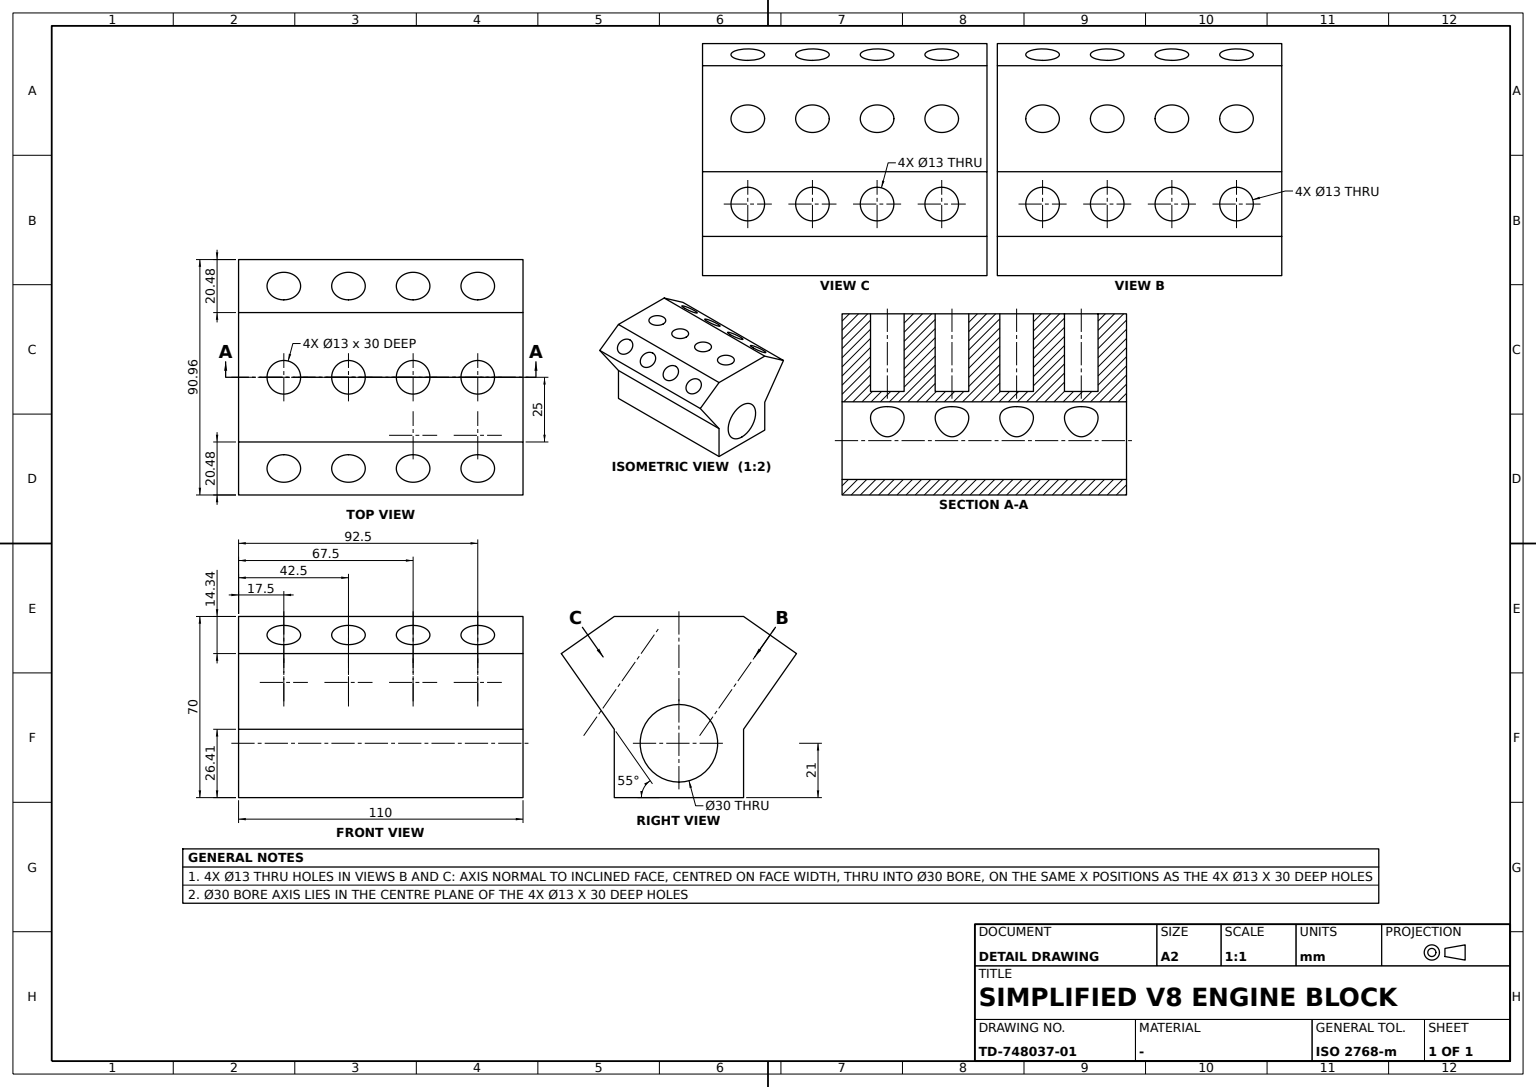
ISO-10303-21;
HEADER;
FILE_DESCRIPTION((''),'2;1');
FILE_NAME('','',(''),(''),'','','');
FILE_SCHEMA(('AUTOMOTIVE_DESIGN'));
ENDSEC;
DATA;
#1=APPLICATION_CONTEXT('');
#2=PRODUCT_CONTEXT('',#1,'mechanical');
#3=PRODUCT('','','',(#2));
#4=PRODUCT_DEFINITION_FORMATION('','',#3);
#5=PRODUCT_DEFINITION_CONTEXT('',#1,'design');
#6=PRODUCT_DEFINITION('','',#4,#5);
#7=PRODUCT_DEFINITION_SHAPE('','',#6);
#8=(LENGTH_UNIT()NAMED_UNIT(*)SI_UNIT(.MILLI.,.METRE.));
#9=(NAMED_UNIT(*)PLANE_ANGLE_UNIT()SI_UNIT($,.RADIAN.));
#10=(NAMED_UNIT(*)SI_UNIT($,.STERADIAN.)SOLID_ANGLE_UNIT());
#11=UNCERTAINTY_MEASURE_WITH_UNIT(LENGTH_MEASURE(0.005),#8,'distance_accuracy_value','');
#12=(GEOMETRIC_REPRESENTATION_CONTEXT(3)GLOBAL_UNCERTAINTY_ASSIGNED_CONTEXT((#11))GLOBAL_UNIT_ASSIGNED_CONTEXT((#8,#9,#10))REPRESENTATION_CONTEXT('',''));
#13=CARTESIAN_POINT('',(11.,-12.129513,29.824676));
#14=VERTEX_POINT('',#13);
#15=CARTESIAN_POINT('',(11.331638,-13.567226,27.566825));
#16=CARTESIAN_POINT('',(10.831406,-12.200834,29.868851));
#17=CARTESIAN_POINT('',(11.342736,-10.406518,31.905828));
#18=CARTESIAN_POINT('',(13.425697,-8.035123,33.778753));
#19=CARTESIAN_POINT('',(18.017567,-6.520434,34.487409));
#20=CARTESIAN_POINT('',(22.326173,-8.58199,33.456222));
#21=CARTESIAN_POINT('',(23.956477,-11.040954,31.272985));
#22=CARTESIAN_POINT('',(24.098074,-12.732658,29.08519));
#23=CARTESIAN_POINT('',(23.306824,-13.919542,26.765346));
#24=CARTESIAN_POINT('',(21.825814,-14.611855,24.598701));
#25=CARTESIAN_POINT('',(19.755642,-14.903136,22.838252));
#26=CARTESIAN_POINT('',(16.99593,-14.94974,22.2127));
#27=CARTESIAN_POINT('',(14.451282,-14.839464,23.383385));
#28=CARTESIAN_POINT('',(12.594119,-14.423445,25.313733));
#29=B_SPLINE_CURVE_WITH_KNOTS('',3,(#15,#16,#17,#18,#19,#20,#21,#22,#23,#24,#25,#26,#27,#28,#15,#16,#17),.UNSPECIFIED.,.T.,.F.,(1,1,1,1,1,1,1,1,1,1,1,1,1,1,1,1,1,1,1,1,1),(-0.008032053,-0.005354702,-0.002677351,0.,0.002677351,0.005354702,0.010709404,0.016064107,0.018741458,0.021418809,0.02409616,0.026773511,0.029450862,0.032128213,0.034805564,0.037482915,0.040160267,0.042837618,0.045514969,0.04819232,0.053547022),.UNSPECIFIED.);
#30=EDGE_CURVE('',#14,#14,#29,.T.);
#31=ORIENTED_EDGE('',*,*,#30,.T.);
#32=EDGE_LOOP('',(#31));
#33=FACE_BOUND('',#32,.T.);
#34=CARTESIAN_POINT('',(17.5,-29.914912,66.557263));
#35=VERTEX_POINT('',#34);
#36=CARTESIAN_POINT('',(17.5,-35.239401,62.829016));
#37=DIRECTION('',(0.,0.573576436,-0.819152044));
#38=DIRECTION('',(0.,0.819152044,0.573576436));
#39=AXIS2_PLACEMENT_3D('',#36,#37,#38);
#40=CIRCLE('',#39,6.5);
#41=EDGE_CURVE('',#35,#35,#40,.T.);
#42=ORIENTED_EDGE('',*,*,#41,.F.);
#43=EDGE_LOOP('',(#42));
#44=FACE_BOUND('',#43,.T.);
#45=CARTESIAN_POINT('',(17.5,-3.283467,17.191213));
#46=DIRECTION('',(-1.,0.,0.));
#47=AXIS2_PLACEMENT_3D('',#45,#37,#46);
#48=CYLINDRICAL_SURFACE('',#47,6.5);
#49=ADVANCED_FACE('',(#33,#44),#48,.F.);
#50=CARTESIAN_POINT('',(24.,12.129513,29.824676));
#51=VERTEX_POINT('',#50);
#52=CARTESIAN_POINT('',(23.655254,10.402376,31.909925));
#53=CARTESIAN_POINT('',(24.169445,12.201153,29.869133));
#54=CARTESIAN_POINT('',(23.666966,13.570089,27.561601));
#55=CARTESIAN_POINT('',(22.399301,14.425934,25.305088));
#56=CARTESIAN_POINT('',(20.543939,14.839822,23.379841));
#57=CARTESIAN_POINT('',(17.996344,14.949835,22.211813));
#58=CARTESIAN_POINT('',(15.240789,14.902833,22.841055));
#59=CARTESIAN_POINT('',(13.173241,14.611379,24.600066));
#60=CARTESIAN_POINT('',(11.692868,13.919632,26.765493));
#61=CARTESIAN_POINT('',(10.904365,12.732991,29.082723));
#62=CARTESIAN_POINT('',(11.037993,11.056515,31.256057));
#63=CARTESIAN_POINT('',(12.666972,8.58389,33.457391));
#64=CARTESIAN_POINT('',(16.974637,6.521635,34.486021));
#65=CARTESIAN_POINT('',(21.569199,8.031851,33.78052));
#66=B_SPLINE_CURVE_WITH_KNOTS('',3,(#52,#53,#54,#55,#56,#57,#58,#59,#60,#61,#62,#63,#64,#65,#52,#53,#54),.UNSPECIFIED.,.T.,.F.,(1,1,1,1,1,1,1,1,1,1,1,1,1,1,1,1,1,1,1,1,1),(-0.010684726,-0.005342363,-0.002671181,0.,0.002671181,0.005342363,0.008013544,0.010684726,0.013355907,0.016027089,0.01869827,0.021369452,0.024040633,0.026711815,0.032054178,0.037396541,0.040067722,0.042738904,0.045410085,0.048081267,0.050752448),.UNSPECIFIED.);
#67=EDGE_CURVE('',#51,#51,#66,.T.);
#68=ORIENTED_EDGE('',*,*,#67,.F.);
#69=EDGE_LOOP('',(#68));
#70=FACE_BOUND('',#69,.T.);
#71=CARTESIAN_POINT('',(17.5,29.914912,66.557263));
#72=VERTEX_POINT('',#71);
#73=CARTESIAN_POINT('',(17.5,35.239401,62.829016));
#74=DIRECTION('',(0.,0.573576436,0.819152044));
#75=DIRECTION('',(0.,-0.819152044,0.573576436));
#76=AXIS2_PLACEMENT_3D('',#73,#74,#75);
#77=CIRCLE('',#76,6.5);
#78=EDGE_CURVE('',#72,#72,#77,.T.);
#79=ORIENTED_EDGE('',*,*,#78,.T.);
#80=EDGE_LOOP('',(#79));
#81=FACE_BOUND('',#80,.T.);
#82=CARTESIAN_POINT('',(17.5,3.283467,17.191213));
#83=AXIS2_PLACEMENT_3D('',#82,#74,#46);
#84=CYLINDRICAL_SURFACE('',#83,6.5);
#85=ADVANCED_FACE('',(#70,#81),#84,.F.);
#86=CARTESIAN_POINT('',(24.,0.,39.998722));
#87=VERTEX_POINT('',#86);
#88=CARTESIAN_POINT('',(17.5,0.,39.998722));
#89=DIRECTION('',(0.,0.,1.));
#90=DIRECTION('',(1.,0.,0.));
#91=AXIS2_PLACEMENT_3D('',#88,#89,#90);
#92=CIRCLE('',#91,6.5);
#93=EDGE_CURVE('',#87,#87,#92,.T.);
#94=ORIENTED_EDGE('',*,*,#93,.T.);
#95=EDGE_LOOP('',(#94));
#96=FACE_BOUND('',#95,.T.);
#97=CARTESIAN_POINT('',(0.,0.,39.998722));
#98=AXIS2_PLACEMENT_3D('',#97,#89,#90);
#99=PLANE('',#98);
#100=ADVANCED_FACE('',(#96),#99,.T.);
#101=CARTESIAN_POINT('',(86.,0.,69.998722));
#102=VERTEX_POINT('',#101);
#103=CARTESIAN_POINT('',(92.5,0.,69.998722));
#104=DIRECTION('',(0.,0.,-1.));
#105=AXIS2_PLACEMENT_3D('',#103,#104,#46);
#106=CIRCLE('',#105,6.5);
#107=EDGE_CURVE('',#102,#102,#106,.F.);
#108=ORIENTED_EDGE('',*,*,#107,.T.);
#109=EDGE_LOOP('',(#108));
#110=FACE_BOUND('',#109,.T.);
#111=CARTESIAN_POINT('',(99.,0.,39.998722));
#112=VERTEX_POINT('',#111);
#113=CARTESIAN_POINT('',(92.5,0.,39.998722));
#114=AXIS2_PLACEMENT_3D('',#113,#89,#90);
#115=CIRCLE('',#114,6.5);
#116=EDGE_CURVE('',#112,#112,#115,.T.);
#117=ORIENTED_EDGE('',*,*,#116,.F.);
#118=EDGE_LOOP('',(#117));
#119=FACE_BOUND('',#118,.T.);
#120=CARTESIAN_POINT('',(92.5,0.,54.998722));
#121=AXIS2_PLACEMENT_3D('',#120,#89,#90);
#122=CYLINDRICAL_SURFACE('',#121,6.5);
#123=ADVANCED_FACE('',(#110,#119),#122,.F.);
#124=CARTESIAN_POINT('',(36.,-12.129513,29.824676));
#125=VERTEX_POINT('',#124);
#126=CARTESIAN_POINT('',(36.331638,-13.567226,27.566825));
#127=CARTESIAN_POINT('',(35.831406,-12.200834,29.868851));
#128=CARTESIAN_POINT('',(36.342736,-10.406518,31.905828));
#129=CARTESIAN_POINT('',(38.425697,-8.035123,33.778753));
#130=CARTESIAN_POINT('',(43.017567,-6.520434,34.487409));
#131=CARTESIAN_POINT('',(47.326173,-8.58199,33.456222));
#132=CARTESIAN_POINT('',(48.956477,-11.040954,31.272985));
#133=CARTESIAN_POINT('',(49.098074,-12.732658,29.08519));
#134=CARTESIAN_POINT('',(48.306824,-13.919542,26.765346));
#135=CARTESIAN_POINT('',(46.825814,-14.611855,24.598701));
#136=CARTESIAN_POINT('',(44.755642,-14.903136,22.838252));
#137=CARTESIAN_POINT('',(41.99593,-14.94974,22.2127));
#138=CARTESIAN_POINT('',(39.451282,-14.839464,23.383385));
#139=CARTESIAN_POINT('',(37.594119,-14.423445,25.313733));
#140=B_SPLINE_CURVE_WITH_KNOTS('',3,(#126,#127,#128,#129,#130,#131,#132,#133,#134,#135,#136,#137,#138,#139,#126,#127,#128),.UNSPECIFIED.,.T.,.F.,(1,1,1,1,1,1,1,1,1,1,1,1,1,1,1,1,1,1,1,1,1),(-0.008032053,-0.005354702,-0.002677351,0.,0.002677351,0.005354702,0.010709404,0.016064107,0.018741458,0.021418809,0.02409616,0.026773511,0.029450862,0.032128213,0.034805564,0.037482915,0.040160267,0.042837618,0.045514969,0.04819232,0.053547022),.UNSPECIFIED.);
#141=EDGE_CURVE('',#125,#125,#140,.T.);
#142=ORIENTED_EDGE('',*,*,#141,.T.);
#143=EDGE_LOOP('',(#142));
#144=FACE_BOUND('',#143,.T.);
#145=CARTESIAN_POINT('',(42.5,-29.914912,66.557263));
#146=VERTEX_POINT('',#145);
#147=CARTESIAN_POINT('',(42.5,-35.239401,62.829016));
#148=AXIS2_PLACEMENT_3D('',#147,#37,#38);
#149=CIRCLE('',#148,6.5);
#150=EDGE_CURVE('',#146,#146,#149,.T.);
#151=ORIENTED_EDGE('',*,*,#150,.F.);
#152=EDGE_LOOP('',(#151));
#153=FACE_BOUND('',#152,.T.);
#154=CARTESIAN_POINT('',(42.5,-3.283467,17.191213));
#155=AXIS2_PLACEMENT_3D('',#154,#37,#46);
#156=CYLINDRICAL_SURFACE('',#155,6.5);
#157=ADVANCED_FACE('',(#144,#153),#156,.F.);
#158=ORIENTED_EDGE('',*,*,#41,.T.);
#159=EDGE_LOOP('',(#158));
#160=FACE_BOUND('',#159,.T.);
#161=CARTESIAN_POINT('',(0.,-45.48,55.658471));
#162=VERTEX_POINT('',#161);
#163=CARTESIAN_POINT('',(110.,-45.48,55.658471));
#164=VERTEX_POINT('',#163);
#165=VECTOR('',#90,1000.);
#166=LINE('',#161,#165);
#167=EDGE_CURVE('',#162,#164,#166,.T.);
#168=ORIENTED_EDGE('',*,*,#167,.T.);
#169=CARTESIAN_POINT('',(110.,-25.,69.998722));
#170=VERTEX_POINT('',#169);
#171=CARTESIAN_POINT('',(110.,-41.113389,58.716005));
#172=VECTOR('',#38,1000.);
#173=LINE('',#171,#172);
#174=EDGE_CURVE('',#164,#170,#173,.T.);
#175=ORIENTED_EDGE('',*,*,#174,.T.);
#176=CARTESIAN_POINT('',(0.,-25.,69.998722));
#177=VERTEX_POINT('',#176);
#178=LINE('',#176,#165);
#179=EDGE_CURVE('',#177,#170,#178,.T.);
#180=ORIENTED_EDGE('',*,*,#179,.F.);
#181=CARTESIAN_POINT('',(0.,-41.113389,58.716005));
#182=LINE('',#181,#172);
#183=EDGE_CURVE('',#162,#177,#182,.T.);
#184=ORIENTED_EDGE('',*,*,#183,.F.);
#185=EDGE_LOOP('',(#168,#175,#180,#184));
#186=FACE_BOUND('',#185,.T.);
#187=CARTESIAN_POINT('',(92.5,-29.914912,66.557263));
#188=VERTEX_POINT('',#187);
#189=CARTESIAN_POINT('',(92.5,-35.239401,62.829016));
#190=AXIS2_PLACEMENT_3D('',#189,#37,#38);
#191=CIRCLE('',#190,6.5);
#192=EDGE_CURVE('',#188,#188,#191,.T.);
#193=ORIENTED_EDGE('',*,*,#192,.T.);
#194=EDGE_LOOP('',(#193));
#195=FACE_BOUND('',#194,.T.);
#196=CARTESIAN_POINT('',(67.5,-29.914912,66.557263));
#197=VERTEX_POINT('',#196);
#198=CARTESIAN_POINT('',(67.5,-35.239401,62.829016));
#199=AXIS2_PLACEMENT_3D('',#198,#37,#38);
#200=CIRCLE('',#199,6.5);
#201=EDGE_CURVE('',#197,#197,#200,.T.);
#202=ORIENTED_EDGE('',*,*,#201,.T.);
#203=EDGE_LOOP('',(#202));
#204=FACE_BOUND('',#203,.T.);
#205=ORIENTED_EDGE('',*,*,#150,.T.);
#206=EDGE_LOOP('',(#205));
#207=FACE_BOUND('',#206,.T.);
#208=AXIS2_PLACEMENT_3D('',#161,#37,#38);
#209=PLANE('',#208);
#210=ADVANCED_FACE('',(#160,#186,#195,#204,#207),#209,.F.);
#211=ORIENTED_EDGE('',*,*,#192,.F.);
#212=EDGE_LOOP('',(#211));
#213=FACE_BOUND('',#212,.T.);
#214=CARTESIAN_POINT('',(99.,-12.129513,29.824676));
#215=VERTEX_POINT('',#214);
#216=CARTESIAN_POINT('',(98.655254,-10.402376,31.909925));
#217=CARTESIAN_POINT('',(99.169445,-12.201153,29.869133));
#218=CARTESIAN_POINT('',(98.666966,-13.570089,27.561601));
#219=CARTESIAN_POINT('',(97.399301,-14.425934,25.305088));
#220=CARTESIAN_POINT('',(95.543939,-14.839822,23.379841));
#221=CARTESIAN_POINT('',(92.996344,-14.949835,22.211813));
#222=CARTESIAN_POINT('',(90.240789,-14.902833,22.841055));
#223=CARTESIAN_POINT('',(88.173241,-14.611379,24.600066));
#224=CARTESIAN_POINT('',(86.692868,-13.919632,26.765493));
#225=CARTESIAN_POINT('',(85.904365,-12.732991,29.082723));
#226=CARTESIAN_POINT('',(86.037993,-11.056515,31.256057));
#227=CARTESIAN_POINT('',(87.666972,-8.58389,33.457391));
#228=CARTESIAN_POINT('',(91.974637,-6.521635,34.486021));
#229=CARTESIAN_POINT('',(96.569199,-8.031851,33.78052));
#230=B_SPLINE_CURVE_WITH_KNOTS('',3,(#216,#217,#218,#219,#220,#221,#222,#223,#224,#225,#226,#227,#228,#229,#216,#217,#218),.UNSPECIFIED.,.T.,.F.,(1,1,1,1,1,1,1,1,1,1,1,1,1,1,1,1,1,1,1,1,1),(-0.010684726,-0.005342363,-0.002671181,0.,0.002671181,0.005342363,0.008013544,0.010684726,0.013355907,0.016027089,0.01869827,0.021369452,0.024040633,0.026711815,0.032054178,0.037396541,0.040067722,0.042738904,0.045410085,0.048081267,0.050752448),.UNSPECIFIED.);
#231=EDGE_CURVE('',#215,#215,#230,.T.);
#232=ORIENTED_EDGE('',*,*,#231,.T.);
#233=EDGE_LOOP('',(#232));
#234=FACE_BOUND('',#233,.T.);
#235=CARTESIAN_POINT('',(92.5,-3.283467,17.191213));
#236=AXIS2_PLACEMENT_3D('',#235,#37,#46);
#237=CYLINDRICAL_SURFACE('',#236,6.5);
#238=ADVANCED_FACE('',(#213,#234),#237,.F.);
#239=ORIENTED_EDGE('',*,*,#116,.T.);
#240=EDGE_LOOP('',(#239));
#241=FACE_BOUND('',#240,.T.);
#242=ADVANCED_FACE('',(#241),#99,.T.);
#243=CARTESIAN_POINT('',(74.,0.,39.998722));
#244=VERTEX_POINT('',#243);
#245=CARTESIAN_POINT('',(67.5,0.,39.998722));
#246=AXIS2_PLACEMENT_3D('',#245,#89,#90);
#247=CIRCLE('',#246,6.5);
#248=EDGE_CURVE('',#244,#244,#247,.T.);
#249=ORIENTED_EDGE('',*,*,#248,.T.);
#250=EDGE_LOOP('',(#249));
#251=FACE_BOUND('',#250,.T.);
#252=ADVANCED_FACE('',(#251),#99,.T.);
#253=ORIENTED_EDGE('',*,*,#248,.F.);
#254=EDGE_LOOP('',(#253));
#255=FACE_BOUND('',#254,.T.);
#256=CARTESIAN_POINT('',(61.,0.,69.998722));
#257=VERTEX_POINT('',#256);
#258=CARTESIAN_POINT('',(67.5,0.,69.998722));
#259=AXIS2_PLACEMENT_3D('',#258,#104,#46);
#260=CIRCLE('',#259,6.5);
#261=EDGE_CURVE('',#257,#257,#260,.F.);
#262=ORIENTED_EDGE('',*,*,#261,.T.);
#263=EDGE_LOOP('',(#262));
#264=FACE_BOUND('',#263,.T.);
#265=CARTESIAN_POINT('',(67.5,0.,54.998722));
#266=AXIS2_PLACEMENT_3D('',#265,#89,#90);
#267=CYLINDRICAL_SURFACE('',#266,6.5);
#268=ADVANCED_FACE('',(#255,#264),#267,.F.);
#269=CARTESIAN_POINT('',(0.,25.,26.41));
#270=VERTEX_POINT('',#269);
#271=CARTESIAN_POINT('',(110.,25.,26.41));
#272=VERTEX_POINT('',#271);
#273=LINE('',#269,#165);
#274=EDGE_CURVE('',#270,#272,#273,.T.);
#275=ORIENTED_EDGE('',*,*,#274,.F.);
#276=CARTESIAN_POINT('',(0.,45.48,55.658471));
#277=VERTEX_POINT('',#276);
#278=CARTESIAN_POINT('',(0.,4.366611,-3.057534));
#279=VECTOR('',#74,1000.);
#280=LINE('',#278,#279);
#281=EDGE_CURVE('',#270,#277,#280,.T.);
#282=ORIENTED_EDGE('',*,*,#281,.T.);
#283=CARTESIAN_POINT('',(110.,45.48,55.658471));
#284=VERTEX_POINT('',#283);
#285=LINE('',#276,#165);
#286=EDGE_CURVE('',#277,#284,#285,.T.);
#287=ORIENTED_EDGE('',*,*,#286,.T.);
#288=CARTESIAN_POINT('',(110.,4.366611,-3.057534));
#289=LINE('',#288,#279);
#290=EDGE_CURVE('',#272,#284,#289,.T.);
#291=ORIENTED_EDGE('',*,*,#290,.F.);
#292=EDGE_LOOP('',(#275,#282,#287,#291));
#293=FACE_BOUND('',#292,.T.);
#294=DIRECTION('',(0.,0.819152044,-0.573576436));
#295=AXIS2_PLACEMENT_3D('',#269,#294,#74);
#296=PLANE('',#295);
#297=ADVANCED_FACE('',(#293),#296,.T.);
#298=CARTESIAN_POINT('',(110.,-25.,0.));
#299=VERTEX_POINT('',#298);
#300=CARTESIAN_POINT('',(110.,25.,0.));
#301=VERTEX_POINT('',#300);
#302=CARTESIAN_POINT('',(110.,0.,0.));
#303=DIRECTION('',(0.,1.,0.));
#304=VECTOR('',#303,1000.);
#305=LINE('',#302,#304);
#306=EDGE_CURVE('',#299,#301,#305,.T.);
#307=ORIENTED_EDGE('',*,*,#306,.F.);
#308=CARTESIAN_POINT('',(0.,-25.,0.));
#309=VERTEX_POINT('',#308);
#310=LINE('',#308,#165);
#311=EDGE_CURVE('',#309,#299,#310,.T.);
#312=ORIENTED_EDGE('',*,*,#311,.F.);
#313=CARTESIAN_POINT('',(0.,25.,0.));
#314=VERTEX_POINT('',#313);
#315=CARTESIAN_POINT('',(0.,0.,0.));
#316=LINE('',#315,#304);
#317=EDGE_CURVE('',#309,#314,#316,.T.);
#318=ORIENTED_EDGE('',*,*,#317,.T.);
#319=LINE('',#313,#165);
#320=EDGE_CURVE('',#314,#301,#319,.T.);
#321=ORIENTED_EDGE('',*,*,#320,.T.);
#322=EDGE_LOOP('',(#307,#312,#318,#321));
#323=FACE_BOUND('',#322,.T.);
#324=AXIS2_PLACEMENT_3D('',#308,#104,#303);
#325=PLANE('',#324);
#326=ADVANCED_FACE('',(#323),#325,.T.);
#327=CARTESIAN_POINT('',(49.,0.,39.998722));
#328=VERTEX_POINT('',#327);
#329=CARTESIAN_POINT('',(42.5,0.,39.998722));
#330=AXIS2_PLACEMENT_3D('',#329,#89,#90);
#331=CIRCLE('',#330,6.5);
#332=EDGE_CURVE('',#328,#328,#331,.T.);
#333=ORIENTED_EDGE('',*,*,#332,.F.);
#334=EDGE_LOOP('',(#333));
#335=FACE_BOUND('',#334,.T.);
#336=CARTESIAN_POINT('',(36.,0.,69.998722));
#337=VERTEX_POINT('',#336);
#338=CARTESIAN_POINT('',(42.5,0.,69.998722));
#339=AXIS2_PLACEMENT_3D('',#338,#104,#46);
#340=CIRCLE('',#339,6.5);
#341=EDGE_CURVE('',#337,#337,#340,.F.);
#342=ORIENTED_EDGE('',*,*,#341,.T.);
#343=EDGE_LOOP('',(#342));
#344=FACE_BOUND('',#343,.T.);
#345=CARTESIAN_POINT('',(42.5,0.,54.998722));
#346=AXIS2_PLACEMENT_3D('',#345,#89,#90);
#347=CYLINDRICAL_SURFACE('',#346,6.5);
#348=ADVANCED_FACE('',(#335,#344),#347,.F.);
#349=CARTESIAN_POINT('',(92.5,29.914912,66.557263));
#350=VERTEX_POINT('',#349);
#351=CARTESIAN_POINT('',(92.5,35.239401,62.829016));
#352=AXIS2_PLACEMENT_3D('',#351,#74,#75);
#353=CIRCLE('',#352,6.5);
#354=EDGE_CURVE('',#350,#350,#353,.T.);
#355=ORIENTED_EDGE('',*,*,#354,.T.);
#356=EDGE_LOOP('',(#355));
#357=FACE_BOUND('',#356,.T.);
#358=CARTESIAN_POINT('',(99.,12.129513,29.824676));
#359=VERTEX_POINT('',#358);
#360=CARTESIAN_POINT('',(98.655254,10.402376,31.909925));
#361=CARTESIAN_POINT('',(99.169445,12.201153,29.869133));
#362=CARTESIAN_POINT('',(98.666966,13.570089,27.561601));
#363=CARTESIAN_POINT('',(97.399301,14.425934,25.305088));
#364=CARTESIAN_POINT('',(95.543939,14.839822,23.379841));
#365=CARTESIAN_POINT('',(92.996344,14.949835,22.211813));
#366=CARTESIAN_POINT('',(90.240789,14.902833,22.841055));
#367=CARTESIAN_POINT('',(88.173241,14.611379,24.600066));
#368=CARTESIAN_POINT('',(86.692868,13.919632,26.765493));
#369=CARTESIAN_POINT('',(85.904365,12.732991,29.082723));
#370=CARTESIAN_POINT('',(86.037993,11.056515,31.256057));
#371=CARTESIAN_POINT('',(87.666972,8.58389,33.457391));
#372=CARTESIAN_POINT('',(91.974637,6.521635,34.486021));
#373=CARTESIAN_POINT('',(96.569199,8.031851,33.78052));
#374=B_SPLINE_CURVE_WITH_KNOTS('',3,(#360,#361,#362,#363,#364,#365,#366,#367,#368,#369,#370,#371,#372,#373,#360,#361,#362),.UNSPECIFIED.,.T.,.F.,(1,1,1,1,1,1,1,1,1,1,1,1,1,1,1,1,1,1,1,1,1),(-0.010684726,-0.005342363,-0.002671181,0.,0.002671181,0.005342363,0.008013544,0.010684726,0.013355907,0.016027089,0.01869827,0.021369452,0.024040633,0.026711815,0.032054178,0.037396541,0.040067722,0.042738904,0.045410085,0.048081267,0.050752448),.UNSPECIFIED.);
#375=EDGE_CURVE('',#359,#359,#374,.T.);
#376=ORIENTED_EDGE('',*,*,#375,.F.);
#377=EDGE_LOOP('',(#376));
#378=FACE_BOUND('',#377,.T.);
#379=CARTESIAN_POINT('',(92.5,3.283467,17.191213));
#380=AXIS2_PLACEMENT_3D('',#379,#74,#46);
#381=CYLINDRICAL_SURFACE('',#380,6.5);
#382=ADVANCED_FACE('',(#357,#378),#381,.F.);
#383=ORIENTED_EDGE('',*,*,#311,.T.);
#384=CARTESIAN_POINT('',(110.,-25.,26.41));
#385=VERTEX_POINT('',#384);
#386=VECTOR('',#89,1000.);
#387=LINE('',#298,#386);
#388=EDGE_CURVE('',#299,#385,#387,.T.);
#389=ORIENTED_EDGE('',*,*,#388,.T.);
#390=CARTESIAN_POINT('',(0.,-25.,26.41));
#391=VERTEX_POINT('',#390);
#392=LINE('',#390,#165);
#393=EDGE_CURVE('',#391,#385,#392,.T.);
#394=ORIENTED_EDGE('',*,*,#393,.F.);
#395=LINE('',#308,#386);
#396=EDGE_CURVE('',#309,#391,#395,.T.);
#397=ORIENTED_EDGE('',*,*,#396,.F.);
#398=EDGE_LOOP('',(#383,#389,#394,#397));
#399=FACE_BOUND('',#398,.T.);
#400=AXIS2_PLACEMENT_3D('',#308,#303,#89);
#401=PLANE('',#400);
#402=ADVANCED_FACE('',(#399),#401,.F.);
#403=ORIENTED_EDGE('',*,*,#274,.T.);
#404=LINE('',#300,#386);
#405=EDGE_CURVE('',#301,#272,#404,.T.);
#406=ORIENTED_EDGE('',*,*,#405,.F.);
#407=ORIENTED_EDGE('',*,*,#320,.F.);
#408=LINE('',#313,#386);
#409=EDGE_CURVE('',#314,#270,#408,.T.);
#410=ORIENTED_EDGE('',*,*,#409,.T.);
#411=EDGE_LOOP('',(#403,#406,#407,#410));
#412=FACE_BOUND('',#411,.T.);
#413=AXIS2_PLACEMENT_3D('',#313,#303,#89);
#414=PLANE('',#413);
#415=ADVANCED_FACE('',(#412),#414,.T.);
#416=CARTESIAN_POINT('',(74.,12.129513,29.824676));
#417=VERTEX_POINT('',#416);
#418=CARTESIAN_POINT('',(73.655254,10.402376,31.909925));
#419=CARTESIAN_POINT('',(74.169445,12.201153,29.869133));
#420=CARTESIAN_POINT('',(73.666966,13.570089,27.561601));
#421=CARTESIAN_POINT('',(72.399301,14.425934,25.305088));
#422=CARTESIAN_POINT('',(70.543939,14.839822,23.379841));
#423=CARTESIAN_POINT('',(67.996344,14.949835,22.211813));
#424=CARTESIAN_POINT('',(65.240789,14.902833,22.841055));
#425=CARTESIAN_POINT('',(63.173241,14.611379,24.600066));
#426=CARTESIAN_POINT('',(61.692868,13.919632,26.765493));
#427=CARTESIAN_POINT('',(60.904365,12.732991,29.082723));
#428=CARTESIAN_POINT('',(61.037993,11.056515,31.256057));
#429=CARTESIAN_POINT('',(62.666972,8.58389,33.457391));
#430=CARTESIAN_POINT('',(66.974637,6.521635,34.486021));
#431=CARTESIAN_POINT('',(71.569199,8.031851,33.78052));
#432=B_SPLINE_CURVE_WITH_KNOTS('',3,(#418,#419,#420,#421,#422,#423,#424,#425,#426,#427,#428,#429,#430,#431,#418,#419,#420),.UNSPECIFIED.,.T.,.F.,(1,1,1,1,1,1,1,1,1,1,1,1,1,1,1,1,1,1,1,1,1),(-0.010684726,-0.005342363,-0.002671181,0.,0.002671181,0.005342363,0.008013544,0.010684726,0.013355907,0.016027089,0.01869827,0.021369452,0.024040633,0.026711815,0.032054178,0.037396541,0.040067722,0.042738904,0.045410085,0.048081267,0.050752448),.UNSPECIFIED.);
#433=EDGE_CURVE('',#417,#417,#432,.T.);
#434=ORIENTED_EDGE('',*,*,#433,.F.);
#435=EDGE_LOOP('',(#434));
#436=FACE_BOUND('',#435,.T.);
#437=CARTESIAN_POINT('',(67.5,29.914912,66.557263));
#438=VERTEX_POINT('',#437);
#439=CARTESIAN_POINT('',(67.5,35.239401,62.829016));
#440=AXIS2_PLACEMENT_3D('',#439,#74,#75);
#441=CIRCLE('',#440,6.5);
#442=EDGE_CURVE('',#438,#438,#441,.T.);
#443=ORIENTED_EDGE('',*,*,#442,.T.);
#444=EDGE_LOOP('',(#443));
#445=FACE_BOUND('',#444,.T.);
#446=CARTESIAN_POINT('',(67.5,3.283467,17.191213));
#447=AXIS2_PLACEMENT_3D('',#446,#74,#46);
#448=CYLINDRICAL_SURFACE('',#447,6.5);
#449=ADVANCED_FACE('',(#436,#445),#448,.F.);
#450=ORIENTED_EDGE('',*,*,#261,.F.);
#451=EDGE_LOOP('',(#450));
#452=FACE_BOUND('',#451,.T.);
#453=ORIENTED_EDGE('',*,*,#179,.T.);
#454=CARTESIAN_POINT('',(110.,25.,69.998722));
#455=VERTEX_POINT('',#454);
#456=CARTESIAN_POINT('',(110.,0.,69.998722));
#457=LINE('',#456,#304);
#458=EDGE_CURVE('',#170,#455,#457,.T.);
#459=ORIENTED_EDGE('',*,*,#458,.T.);
#460=CARTESIAN_POINT('',(0.,25.,69.998722));
#461=VERTEX_POINT('',#460);
#462=LINE('',#460,#165);
#463=EDGE_CURVE('',#461,#455,#462,.T.);
#464=ORIENTED_EDGE('',*,*,#463,.F.);
#465=CARTESIAN_POINT('',(0.,0.,69.998722));
#466=LINE('',#465,#304);
#467=EDGE_CURVE('',#177,#461,#466,.T.);
#468=ORIENTED_EDGE('',*,*,#467,.F.);
#469=EDGE_LOOP('',(#453,#459,#464,#468));
#470=FACE_BOUND('',#469,.T.);
#471=ORIENTED_EDGE('',*,*,#107,.F.);
#472=EDGE_LOOP('',(#471));
#473=FACE_BOUND('',#472,.T.);
#474=ORIENTED_EDGE('',*,*,#341,.F.);
#475=EDGE_LOOP('',(#474));
#476=FACE_BOUND('',#475,.T.);
#477=CARTESIAN_POINT('',(11.,0.,69.998722));
#478=VERTEX_POINT('',#477);
#479=CARTESIAN_POINT('',(17.5,0.,69.998722));
#480=AXIS2_PLACEMENT_3D('',#479,#104,#46);
#481=CIRCLE('',#480,6.5);
#482=EDGE_CURVE('',#478,#478,#481,.F.);
#483=ORIENTED_EDGE('',*,*,#482,.F.);
#484=EDGE_LOOP('',(#483));
#485=FACE_BOUND('',#484,.T.);
#486=AXIS2_PLACEMENT_3D('',#176,#104,#303);
#487=PLANE('',#486);
#488=ADVANCED_FACE('',(#452,#470,#473,#476,#485),#487,.F.);
#489=ORIENTED_EDGE('',*,*,#482,.T.);
#490=EDGE_LOOP('',(#489));
#491=FACE_BOUND('',#490,.T.);
#492=ORIENTED_EDGE('',*,*,#93,.F.);
#493=EDGE_LOOP('',(#492));
#494=FACE_BOUND('',#493,.T.);
#495=CARTESIAN_POINT('',(17.5,0.,54.998722));
#496=AXIS2_PLACEMENT_3D('',#495,#89,#90);
#497=CYLINDRICAL_SURFACE('',#496,6.5);
#498=ADVANCED_FACE('',(#491,#494),#497,.F.);
#499=ORIENTED_EDGE('',*,*,#67,.T.);
#500=EDGE_LOOP('',(#499));
#501=FACE_BOUND('',#500,.T.);
#502=ORIENTED_EDGE('',*,*,#141,.F.);
#503=EDGE_LOOP('',(#502));
#504=FACE_BOUND('',#503,.T.);
#505=CARTESIAN_POINT('',(0.,0.,6.));
#506=VERTEX_POINT('',#505);
#507=CARTESIAN_POINT('',(0.,0.,21.));
#508=AXIS2_PLACEMENT_3D('',#507,#90,#104);
#509=CIRCLE('',#508,15.);
#510=EDGE_CURVE('',#506,#506,#509,.T.);
#511=ORIENTED_EDGE('',*,*,#510,.F.);
#512=EDGE_LOOP('',(#511));
#513=FACE_BOUND('',#512,.T.);
#514=ORIENTED_EDGE('',*,*,#30,.F.);
#515=EDGE_LOOP('',(#514));
#516=FACE_BOUND('',#515,.T.);
#517=CARTESIAN_POINT('',(61.,-12.129513,29.824676));
#518=VERTEX_POINT('',#517);
#519=CARTESIAN_POINT('',(61.331638,-13.567226,27.566825));
#520=CARTESIAN_POINT('',(60.831406,-12.200834,29.868851));
#521=CARTESIAN_POINT('',(61.342736,-10.406518,31.905828));
#522=CARTESIAN_POINT('',(63.425697,-8.035123,33.778753));
#523=CARTESIAN_POINT('',(68.017567,-6.520434,34.487409));
#524=CARTESIAN_POINT('',(72.326173,-8.58199,33.456222));
#525=CARTESIAN_POINT('',(73.956477,-11.040954,31.272985));
#526=CARTESIAN_POINT('',(74.098074,-12.732658,29.08519));
#527=CARTESIAN_POINT('',(73.306824,-13.919542,26.765346));
#528=CARTESIAN_POINT('',(71.825814,-14.611855,24.598701));
#529=CARTESIAN_POINT('',(69.755642,-14.903136,22.838252));
#530=CARTESIAN_POINT('',(66.99593,-14.94974,22.2127));
#531=CARTESIAN_POINT('',(64.451282,-14.839464,23.383385));
#532=CARTESIAN_POINT('',(62.594119,-14.423445,25.313733));
#533=B_SPLINE_CURVE_WITH_KNOTS('',3,(#519,#520,#521,#522,#523,#524,#525,#526,#527,#528,#529,#530,#531,#532,#519,#520,#521),.UNSPECIFIED.,.T.,.F.,(1,1,1,1,1,1,1,1,1,1,1,1,1,1,1,1,1,1,1,1,1),(-0.008032053,-0.005354702,-0.002677351,0.,0.002677351,0.005354702,0.010709404,0.016064107,0.018741458,0.021418809,0.02409616,0.026773511,0.029450862,0.032128213,0.034805564,0.037482915,0.040160267,0.042837618,0.045514969,0.04819232,0.053547022),.UNSPECIFIED.);
#534=EDGE_CURVE('',#518,#518,#533,.T.);
#535=ORIENTED_EDGE('',*,*,#534,.F.);
#536=EDGE_LOOP('',(#535));
#537=FACE_BOUND('',#536,.T.);
#538=ORIENTED_EDGE('',*,*,#375,.T.);
#539=EDGE_LOOP('',(#538));
#540=FACE_BOUND('',#539,.T.);
#541=ORIENTED_EDGE('',*,*,#231,.F.);
#542=EDGE_LOOP('',(#541));
#543=FACE_BOUND('',#542,.T.);
#544=CARTESIAN_POINT('',(110.,0.,6.));
#545=VERTEX_POINT('',#544);
#546=CARTESIAN_POINT('',(110.,0.,21.));
#547=AXIS2_PLACEMENT_3D('',#546,#90,#104);
#548=CIRCLE('',#547,15.);
#549=EDGE_CURVE('',#545,#545,#548,.T.);
#550=ORIENTED_EDGE('',*,*,#549,.T.);
#551=EDGE_LOOP('',(#550));
#552=FACE_BOUND('',#551,.T.);
#553=ORIENTED_EDGE('',*,*,#433,.T.);
#554=EDGE_LOOP('',(#553));
#555=FACE_BOUND('',#554,.T.);
#556=CARTESIAN_POINT('',(49.,12.129513,29.824676));
#557=VERTEX_POINT('',#556);
#558=CARTESIAN_POINT('',(48.655254,10.402376,31.909925));
#559=CARTESIAN_POINT('',(49.169445,12.201153,29.869133));
#560=CARTESIAN_POINT('',(48.666966,13.570089,27.561601));
#561=CARTESIAN_POINT('',(47.399301,14.425934,25.305088));
#562=CARTESIAN_POINT('',(45.543939,14.839822,23.379841));
#563=CARTESIAN_POINT('',(42.996344,14.949835,22.211813));
#564=CARTESIAN_POINT('',(40.240789,14.902833,22.841055));
#565=CARTESIAN_POINT('',(38.173241,14.611379,24.600066));
#566=CARTESIAN_POINT('',(36.692868,13.919632,26.765493));
#567=CARTESIAN_POINT('',(35.904365,12.732991,29.082723));
#568=CARTESIAN_POINT('',(36.037993,11.056515,31.256057));
#569=CARTESIAN_POINT('',(37.666972,8.58389,33.457391));
#570=CARTESIAN_POINT('',(41.974637,6.521635,34.486021));
#571=CARTESIAN_POINT('',(46.569199,8.031851,33.78052));
#572=B_SPLINE_CURVE_WITH_KNOTS('',3,(#558,#559,#560,#561,#562,#563,#564,#565,#566,#567,#568,#569,#570,#571,#558,#559,#560),.UNSPECIFIED.,.T.,.F.,(1,1,1,1,1,1,1,1,1,1,1,1,1,1,1,1,1,1,1,1,1),(-0.010684726,-0.005342363,-0.002671181,0.,0.002671181,0.005342363,0.008013544,0.010684726,0.013355907,0.016027089,0.01869827,0.021369452,0.024040633,0.026711815,0.032054178,0.037396541,0.040067722,0.042738904,0.045410085,0.048081267,0.050752448),.UNSPECIFIED.);
#573=EDGE_CURVE('',#557,#557,#572,.T.);
#574=ORIENTED_EDGE('',*,*,#573,.T.);
#575=EDGE_LOOP('',(#574));
#576=FACE_BOUND('',#575,.T.);
#577=CARTESIAN_POINT('',(55.,0.,21.));
#578=AXIS2_PLACEMENT_3D('',#577,#90,#303);
#579=CYLINDRICAL_SURFACE('',#578,15.);
#580=ADVANCED_FACE('',(#501,#504,#513,#516,#537,#540,#543,#552,#555,#576),#579,.F.);
#581=ORIENTED_EDGE('',*,*,#549,.F.);
#582=EDGE_LOOP('',(#581));
#583=FACE_BOUND('',#582,.T.);
#584=ORIENTED_EDGE('',*,*,#174,.F.);
#585=CARTESIAN_POINT('',(110.,-4.366611,-3.057534));
#586=DIRECTION('',(0.,-0.573576436,0.819152044));
#587=VECTOR('',#586,1000.);
#588=LINE('',#585,#587);
#589=EDGE_CURVE('',#385,#164,#588,.T.);
#590=ORIENTED_EDGE('',*,*,#589,.F.);
#591=ORIENTED_EDGE('',*,*,#388,.F.);
#592=ORIENTED_EDGE('',*,*,#306,.T.);
#593=ORIENTED_EDGE('',*,*,#405,.T.);
#594=ORIENTED_EDGE('',*,*,#290,.T.);
#595=CARTESIAN_POINT('',(110.,41.113389,58.716005));
#596=VECTOR('',#75,1000.);
#597=LINE('',#595,#596);
#598=EDGE_CURVE('',#284,#455,#597,.T.);
#599=ORIENTED_EDGE('',*,*,#598,.T.);
#600=ORIENTED_EDGE('',*,*,#458,.F.);
#601=EDGE_LOOP('',(#584,#590,#591,#592,#593,#594,#599,#600));
#602=FACE_BOUND('',#601,.T.);
#603=AXIS2_PLACEMENT_3D('',#302,#90,#303);
#604=PLANE('',#603);
#605=ADVANCED_FACE('',(#583,#602),#604,.T.);
#606=ORIENTED_EDGE('',*,*,#332,.T.);
#607=EDGE_LOOP('',(#606));
#608=FACE_BOUND('',#607,.T.);
#609=ADVANCED_FACE('',(#608),#99,.T.);
#610=CARTESIAN_POINT('',(42.5,29.914912,66.557263));
#611=VERTEX_POINT('',#610);
#612=CARTESIAN_POINT('',(42.5,35.239401,62.829016));
#613=AXIS2_PLACEMENT_3D('',#612,#74,#75);
#614=CIRCLE('',#613,6.5);
#615=EDGE_CURVE('',#611,#611,#614,.T.);
#616=ORIENTED_EDGE('',*,*,#615,.T.);
#617=EDGE_LOOP('',(#616));
#618=FACE_BOUND('',#617,.T.);
#619=ORIENTED_EDGE('',*,*,#573,.F.);
#620=EDGE_LOOP('',(#619));
#621=FACE_BOUND('',#620,.T.);
#622=CARTESIAN_POINT('',(42.5,3.283467,17.191213));
#623=AXIS2_PLACEMENT_3D('',#622,#74,#46);
#624=CYLINDRICAL_SURFACE('',#623,6.5);
#625=ADVANCED_FACE('',(#618,#621),#624,.F.);
#626=ORIENTED_EDGE('',*,*,#201,.F.);
#627=EDGE_LOOP('',(#626));
#628=FACE_BOUND('',#627,.T.);
#629=ORIENTED_EDGE('',*,*,#534,.T.);
#630=EDGE_LOOP('',(#629));
#631=FACE_BOUND('',#630,.T.);
#632=CARTESIAN_POINT('',(67.5,-3.283467,17.191213));
#633=AXIS2_PLACEMENT_3D('',#632,#37,#46);
#634=CYLINDRICAL_SURFACE('',#633,6.5);
#635=ADVANCED_FACE('',(#628,#631),#634,.F.);
#636=ORIENTED_EDGE('',*,*,#510,.T.);
#637=EDGE_LOOP('',(#636));
#638=FACE_BOUND('',#637,.T.);
#639=ORIENTED_EDGE('',*,*,#409,.F.);
#640=ORIENTED_EDGE('',*,*,#317,.F.);
#641=ORIENTED_EDGE('',*,*,#396,.T.);
#642=CARTESIAN_POINT('',(0.,-4.366611,-3.057534));
#643=LINE('',#642,#587);
#644=EDGE_CURVE('',#391,#162,#643,.T.);
#645=ORIENTED_EDGE('',*,*,#644,.T.);
#646=ORIENTED_EDGE('',*,*,#183,.T.);
#647=ORIENTED_EDGE('',*,*,#467,.T.);
#648=CARTESIAN_POINT('',(0.,41.113389,58.716005));
#649=LINE('',#648,#596);
#650=EDGE_CURVE('',#277,#461,#649,.T.);
#651=ORIENTED_EDGE('',*,*,#650,.F.);
#652=ORIENTED_EDGE('',*,*,#281,.F.);
#653=EDGE_LOOP('',(#639,#640,#641,#645,#646,#647,#651,#652));
#654=FACE_BOUND('',#653,.T.);
#655=AXIS2_PLACEMENT_3D('',#315,#90,#303);
#656=PLANE('',#655);
#657=ADVANCED_FACE('',(#638,#654),#656,.F.);
#658=ORIENTED_EDGE('',*,*,#354,.F.);
#659=EDGE_LOOP('',(#658));
#660=FACE_BOUND('',#659,.T.);
#661=ORIENTED_EDGE('',*,*,#286,.F.);
#662=ORIENTED_EDGE('',*,*,#650,.T.);
#663=ORIENTED_EDGE('',*,*,#463,.T.);
#664=ORIENTED_EDGE('',*,*,#598,.F.);
#665=EDGE_LOOP('',(#661,#662,#663,#664));
#666=FACE_BOUND('',#665,.T.);
#667=ORIENTED_EDGE('',*,*,#442,.F.);
#668=EDGE_LOOP('',(#667));
#669=FACE_BOUND('',#668,.T.);
#670=ORIENTED_EDGE('',*,*,#78,.F.);
#671=EDGE_LOOP('',(#670));
#672=FACE_BOUND('',#671,.T.);
#673=ORIENTED_EDGE('',*,*,#615,.F.);
#674=EDGE_LOOP('',(#673));
#675=FACE_BOUND('',#674,.T.);
#676=AXIS2_PLACEMENT_3D('',#276,#74,#75);
#677=PLANE('',#676);
#678=ADVANCED_FACE('',(#660,#666,#669,#672,#675),#677,.T.);
#679=ORIENTED_EDGE('',*,*,#589,.T.);
#680=ORIENTED_EDGE('',*,*,#167,.F.);
#681=ORIENTED_EDGE('',*,*,#644,.F.);
#682=ORIENTED_EDGE('',*,*,#393,.T.);
#683=EDGE_LOOP('',(#679,#680,#681,#682));
#684=FACE_BOUND('',#683,.T.);
#685=AXIS2_PLACEMENT_3D('',#390,#38,#586);
#686=PLANE('',#685);
#687=ADVANCED_FACE('',(#684),#686,.F.);
#688=CLOSED_SHELL('',(#49,#85,#100,#123,#157,#210,#238,#242,#252,#268,#297,#326,#348,#382,#402,#415,#449,#488,#498,#580,#605,#609,#625,#635,#657,#678,#687));
#689=MANIFOLD_SOLID_BREP('',#688);
#690=ADVANCED_BREP_SHAPE_REPRESENTATION('',(#689),#12);
#691=SHAPE_DEFINITION_REPRESENTATION(#7,#690);
ENDSEC;
END-ISO-10303-21;
